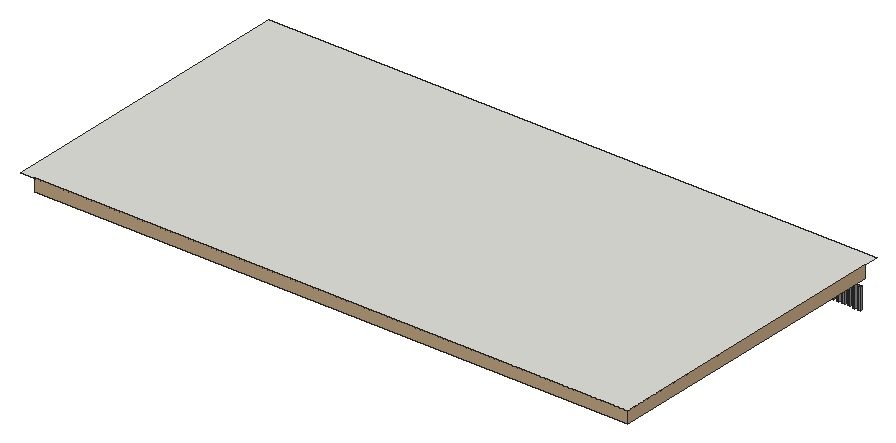
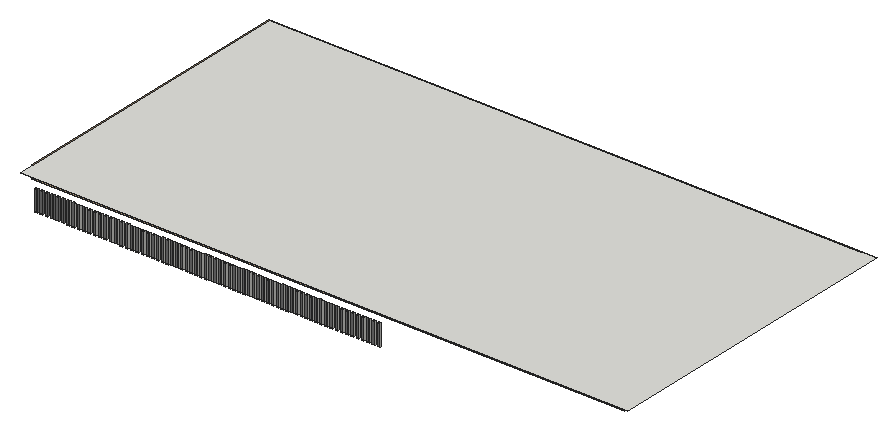
# SketchUp Ruby script. Lengths in inches.
U = 1.inch
M = Sketchup.active_model
def pt(a) = Geom::Point3d.new(a.map { |v| v * U })
def face(e, loops, mat)
  f = e.add_face(loops[0].map { |a| pt(a) })
  loops[1..].each { |l| e.add_face(l.map { |a| pt(a) }).erase! }
  f.material = f.back_material = mat if mat
  f
end
# faces: each face lists its corners as indices into pts; further lists are holes
def faces(e, pts, list, mat = nil) = list.each { |f| face(e, (f[0].is_a?(Array) ? f : [f]).map { |l| l.map { |i| pts[i] } }, mat) }
# xy, xz, yz: faces in a plane at the given z, y or x. An outline is a flat list of corners, or four numbers for a rectangle; further outlines are holes
def ring(l) = l.size == 4 ? [[l[0], l[1]], [l[2], l[1]], [l[2], l[3]], [l[0], l[3]]] : l.each_slice(2).to_a
def flat(e, list, mat, &to3) = list.each { |f| face(e, (f[0].is_a?(Array) ? f : [f]).map { |l| ring(l).map { |u, v| to3.(u, v) } }, mat) }
def xy(e, z, list, mat = nil) = flat(e, list, mat) { |x, y| [x, y, z] }
def xz(e, y, list, mat = nil) = flat(e, list, mat) { |x, z| [x, y, z] }
def yz(e, x, list, mat = nil) = flat(e, list, mat) { |y, z| [x, y, z] }
def lines(e, pts, list) = list.each { |a, b| e.add_line(pt(pts[a]), pt(pts[b])) }
# prism: a flat outline (further loops are holes) pulled along v
def prism(e, loops, v, mat = nil)
  f = face(e, loops, mat); d = Geom::Vector3d.new(v.map { |x| x * U })
  f.pushpull(f.normal.samedirection?(d) ? d.length : -d.length)
end
def box(e, o, s, mat = nil) = prism(e, [[o, [o[0] + s[0], o[1], o[2]], [o[0] + s[0], o[1] + s[1], o[2]], [o[0], o[1] + s[1], o[2]]]], [0, 0, s[2]], mat)
def at(x, y, z, deg = 0) = Geom::Transformation.translation(pt([x, y, z])) * Geom::Transformation.rotation(ORIGIN, Z_AXIS, deg.degrees)
def axes(o, x, y, z) = Geom::Transformation.new([*x, 0, *y, 0, *z, 0, *pt(o).to_a, 1])
def part(name) = M.definitions.add(name)
# library, detail: a bought-in or finely detailed component or shape, given as its bounding box
def library(name, o, s) = part(name).tap { |d| box(d.entities, o, s) }
def detail(e, o, s) = box(e.add_group.entities, o, s)
def put(e, d, t, mat = nil) = e.add_instance(d, t).tap { |i| i.material = mat if mat }
def group(e, t, mat = nil) = e.add_group.tap { |g| g.transformation = t; g.material = mat if mat }.entities
root = M.entities
M.materials.add("Maquette Wood A01 12cm").color = [209, 181, 135]
M.materials.add("Sand A01 200cm").color = [193, 166, 131]
M.materials.add("[Color M04]").color = [142, 142, 142]
c1 = library("Spot Light\#2",[-5.1,-5.1,-11.05],[10.2,10.2,11.05])
c2 = library("Spot Light\#5",[-5.1,-5.1,-11.05],[10.2,10.2,11.05])
c3 = library("Fan 90-20",[-15.86,-15.86,-9.19],[31.73,31.72,9.19])
c4 = library("Spot Light\#1",[-5.1,-5.1,-11.05],[10.2,10.2,11.05])
c5 = library("Spot Light\#6",[-5.1,-5.1,-11.05],[10.2,10.2,11.05])
c6 = library("Spot Light",[-5.1,-5.1,-11.05],[10.2,10.2,11.05])
c7 = library("Spot Light\#7",[-5.1,-5.1,-11.05],[10.2,10.2,11.05])
xy(root,222.8125,[[195.59,222.56,197.53,223.75],[199.5625,222.56,201.5,223.75],[203.53,222.56,205.47,223.75],[207.5,222.56,209.44,223.75],[211.47,222.56,213.41,223.75],
  [215.4375,222.56,217.38,223.75],[219.41,222.56,221.35,223.75],[223.38,222.56,225.32,223.75],[227.35,222.56,229.29,223.75],[231.32,222.56,233.26,223.75],
  [235.29,222.56,237.23,223.75],[239.25,222.56,241.2,223.75],[242.87,222.56,244.8125,223.75],[246.49,222.56,248.43,223.75],[250.11,222.56,252.05,223.75],
  [253.72,222.56,255.67,223.75],[257.34,222.56,259.28,223.75],[260.96,222.56,262.9,223.75],[264.58,222.56,266.52,223.75],[268.19,222.56,270.14,223.75],
  [271.8125,222.56,273.75,223.75],[275.43,222.56,277.37,223.75],[279.05,222.56,280.99,223.75],[282.66,222.56,284.61,223.75],[286.28,222.56,288.22,223.75],
  [289.9,222.56,291.84,223.75],[293.52,222.56,295.46,223.75],[297.13,222.56,299.08,223.75],[300.75,222.56,302.69,223.75],[304.37,222.56,306.31,223.75],
  [307.99,222.56,309.93,223.75],[311.6,222.56,313.55,223.75],[315.22,222.56,317.16,223.75],[318.84,222.56,320.78,223.75],[322.46,222.56,324.4,223.75],
  [326.07,222.56,328.01,223.75],[329.69,222.56,331.63,223.75],[333.31,222.56,335.25,223.75],[336.93,222.56,338.87,223.75],[340.54,222.56,342.48,223.75],
  [344.16,222.56,346.1,223.75],[347.78,222.56,349.72,223.75],[351.39,222.56,353.34,223.75],[355.01,222.56,356.95,223.75],[358.63,222.56,360.57,223.75],
  [362.44,222.56,364.38,223.75],[365.5,222.56,367.45,223.75],[369.54,222.56,371.48,223.75],[373.57,222.56,375.51,223.75],[377.6,222.56,379.54,223.75],
  [381.63,222.56,383.57,223.75],[385.66,222.56,387.6,223.75],[389.69,222.56,391.63,223.75],[393.72,222.56,395.67,223.75],[397.75,222.56,399.7,223.75],
  [401.79,222.56,403.73,223.75],[405.82,222.56,407.76,223.75],[409.85,222.56,411.79,223.75],[413.88,222.56,415.82,223.75],[417.91,222.56,419.85,223.75],
  [421.94,222.56,423.88,223.75],[425.97,222.56,427.92,223.75],[430,222.56,431.95,223.75]])
xy(root,222.8125,[[434.04,222.56,435.98,223.75],[438.07,222.56,440.01,223.75],[442.1,222.56,444.04,223.75],[446.13,222.56,448.07,223.75],[450.16,222.56,452.1,223.75],
  [454.19,222.56,456.13,223.75]],"[Color M04]")
xy(root,238.625,[[329.69,222.56,331.63,223.75],[347.78,222.56,349.72,223.75]])
xy(root,238.625,[[195.59,222.56,197.53,223.75],[199.5625,222.56,201.5,223.75],[203.53,222.56,205.47,223.75],[207.5,222.56,209.44,223.75],[211.47,222.56,213.41,223.75],
  [215.4375,222.56,217.38,223.75],[219.41,222.56,221.35,223.75],[223.38,222.56,225.32,223.75],[227.35,222.56,229.29,223.75],[231.32,222.56,233.26,223.75],
  [235.29,222.56,237.23,223.75],[239.25,222.56,241.2,223.75],[242.87,222.56,244.8125,223.75],[246.49,222.56,248.43,223.75],[250.11,222.56,252.05,223.75],
  [253.72,222.56,255.67,223.75],[257.34,222.56,259.28,223.75],[260.96,222.56,262.9,223.75],[264.58,222.56,266.52,223.75],[268.19,222.56,270.14,223.75],
  [271.8125,222.56,273.75,223.75],[275.43,222.56,277.37,223.75],[279.05,222.56,280.99,223.75],[282.66,222.56,284.61,223.75],[286.28,222.56,288.22,223.75],
  [289.9,222.56,291.84,223.75],[293.52,222.56,295.46,223.75],[297.13,222.56,299.08,223.75],[300.75,222.56,302.69,223.75],[304.37,222.56,306.31,223.75],
  [307.99,222.56,309.93,223.75],[311.6,222.56,313.55,223.75],[315.22,222.56,317.16,223.75],[318.84,222.56,320.78,223.75],[322.46,222.56,324.4,223.75],
  [326.07,222.56,328.01,223.75],[333.31,222.56,335.25,223.75],[336.93,222.56,338.87,223.75],[340.54,222.56,342.48,223.75],[344.16,222.56,346.1,223.75],
  [351.39,222.56,353.34,223.75],[355.01,222.56,356.95,223.75],[358.63,222.56,360.57,223.75],[362.44,222.56,364.38,223.75],[365.5,222.56,367.45,223.75],
  [369.54,222.56,371.48,223.75],[373.57,222.56,375.51,223.75],[377.6,222.56,379.54,223.75],[381.63,222.56,383.57,223.75],[385.66,222.56,387.6,223.75],
  [389.69,222.56,391.63,223.75],[393.72,222.56,395.67,223.75],[397.75,222.56,399.7,223.75],[401.79,222.56,403.73,223.75],[405.82,222.56,407.76,223.75],
  [409.85,222.56,411.79,223.75],[413.88,222.56,415.82,223.75],[417.91,222.56,419.85,223.75],[421.94,222.56,423.88,223.75],[425.97,222.56,427.92,223.75],
  [430,222.56,431.95,223.75],[434.04,222.56,435.98,223.75],[438.07,222.56,440.01,223.75],[442.1,222.56,444.04,223.75],[446.13,222.56,448.07,223.75],
  [450.16,222.56,452.1,223.75],[454.19,222.56,456.13,223.75]],"[Color M04]")
xy(root,240.875,[[[36.86,36.86,432.41,198.01],[119.36,152.06,123.11,152.55,126.61,154,129.61,156.31,131.92,159.31,133.37,162.81,133.86,166.56,133.37,170.3125,131.92,173.81,129.61,176.8125,126.61,179.12,123.11,180.57,119.36,181.06,115.61,180.57,112.11,179.12,109.11,176.8125,106.8,173.81,105.35,170.3125,104.86,166.56,105.35,162.81,106.8,159.31,109.11,156.31,112.11,154,115.61,152.55],[380.67,152.06,384.43,152.55,387.92,154,390.93,156.31,393.23,159.31,394.68,162.81,395.17,166.56,394.68,170.3125,393.23,173.81,390.93,176.8125,387.92,179.12,384.43,180.57,380.67,181.06,376.92,180.57,373.42,179.12,370.42,176.8125,368.12,173.81,366.67,170.3125,366.17,166.56,366.67,162.81,368.12,159.31,370.42,156.31,373.42,154,376.92,152.55],[380.67,56.94,384.43,57.43,387.92,58.88,390.93,61.18,393.23,64.19,394.68,67.68,395.17,71.44,394.68,75.1875,393.23,78.69,390.93,81.6875,387.92,83.99,384.43,85.44,380.67,85.94,376.92,85.44,373.42,83.99,370.42,81.6875,368.12,78.69,366.67,75.1875,366.17,71.44,366.67,67.68,368.12,64.19,370.42,61.18,373.42,58.88,376.92,57.43],[119.36,55.56,123.11,56.05,126.61,57.5,129.61,59.81,131.92,62.81,133.37,66.31,133.86,70.06,133.37,73.8125,131.92,77.31,129.61,80.3125,126.61,82.62,123.11,84.07,119.36,84.56,115.61,84.07,112.11,82.62,109.11,80.3125,106.8,77.31,105.35,73.8125,104.86,70.06,105.35,66.31,106.8,62.81,109.11,59.81,112.11,57.5,115.61,56.05],[286.11,152.34,288.26,152.62,290.27,153.45,291.99,154.77,293.31,156.49,294.14,158.5,294.42,160.65,294.14,162.8,293.31,164.8,291.99,166.53,290.27,167.85,288.26,168.68,286.11,168.96,283.96,168.68,281.95,167.85,280.23,166.53,278.91,164.8,278.08,162.8,277.8,160.65,278.08,158.5,278.91,156.49,280.23,154.77,281.95,153.45,283.96,152.62],[201.74,152.34,203.89,152.62,205.89,153.45,207.61,154.77,208.93,156.49,209.76,158.5,210.05,160.65,209.76,162.8,208.93,164.8,207.61,166.53,205.89,167.85,203.89,168.68,201.74,168.96,199.58,168.68,197.58,167.85,195.86,166.53,194.54,164.8,193.71,162.8,193.42,160.65,193.71,158.5,194.54,156.49,195.86,154.77,197.58,153.45,199.58,152.62],[201.74,60.65,203.89,60.93,205.89,61.76,207.61,63.08,208.93,64.8,209.76,66.81,210.05,68.96,209.76,71.11,208.93,73.12,207.61,74.84,205.89,76.16,203.89,76.99,201.74,77.27,199.58,76.99,197.58,76.16,195.86,74.84,194.54,73.12,193.71,71.11,193.42,68.96,193.71,66.81,194.54,64.8,195.86,63.08,197.58,61.76,199.58,60.93],[286.11,63.4,288.26,63.68,290.27,64.51,291.99,65.83,293.31,67.55,294.14,69.56,294.42,71.71,294.14,73.86,293.31,75.87,291.99,77.59,290.27,78.91,288.26,79.74,286.11,80.02,283.96,79.74,281.95,78.91,280.23,77.59,278.91,75.87,278.08,73.86,277.8,71.71,278.08,69.56,278.91,67.55,280.23,65.83,281.95,64.51,283.96,63.68]]],"[Color M04]")
xy(root,242.375,[[286.11,63.4,283.96,63.68,281.95,64.51,280.23,65.83,278.91,67.55,278.08,69.56,277.8,71.71,278.08,73.86,278.91,75.87,280.23,77.59,281.95,78.91,283.96,79.74,286.11,80.02,288.26,79.74,290.27,78.91,291.99,77.59,293.31,75.87,294.14,73.86,294.42,71.71,294.14,69.56,293.31,67.55,291.99,65.83,290.27,64.51,288.26,63.68]],"[Color M04]")
xy(root,242.5625,[[201.74,60.65,199.58,60.93,197.58,61.76,195.86,63.08,194.54,64.8,193.71,66.81,193.42,68.96,193.71,71.11,194.54,73.12,195.86,74.84,197.58,76.16,199.58,76.99,201.74,77.27,203.89,76.99,205.89,76.16,207.61,74.84,208.93,73.12,209.76,71.11,210.05,68.96,209.76,66.81,208.93,64.8,207.61,63.08,205.89,61.76,203.89,60.93]],"[Color M04]")
xy(root,242.75,[[201.74,152.34,199.58,152.62,197.58,153.45,195.86,154.77,194.54,156.49,193.71,158.5,193.42,160.65,193.71,162.8,194.54,164.8,195.86,166.53,197.58,167.85,199.58,168.68,201.74,168.96,203.89,168.68,205.89,167.85,207.61,166.53,208.93,164.8,209.76,162.8,210.05,160.65,209.76,158.5,208.93,156.49,207.61,154.77,205.89,153.45,203.89,152.62]],"[Color M04]")
xy(root,242.875,[[286.11,152.34,283.96,152.62,281.95,153.45,280.23,154.77,278.91,156.49,278.08,158.5,277.8,160.65,278.08,162.8,278.91,164.8,280.23,166.53,281.95,167.85,283.96,168.68,286.11,168.96,288.26,168.68,290.27,167.85,291.99,166.53,293.31,164.8,294.14,162.8,294.42,160.65,294.14,158.5,293.31,156.49,291.99,154.77,290.27,153.45,288.26,152.62]],"[Color M04]")
xy(root,242.9375,[[380.67,152.06,376.92,152.55,373.42,154,370.42,156.31,368.12,159.31,366.67,162.81,366.17,166.56,366.67,170.3125,368.12,173.81,370.42,176.8125,373.42,179.12,376.92,180.57,380.67,181.06,384.43,180.57,387.92,179.12,390.93,176.8125,393.23,173.81,394.68,170.3125,395.17,166.56,394.68,162.81,393.23,159.31,390.93,156.31,387.92,154,384.43,152.55]],"[Color M04]")
xy(root,243.0625,[[380.67,56.94,376.92,57.43,373.42,58.88,370.42,61.18,368.12,64.19,366.67,67.68,366.17,71.44,366.67,75.1875,368.12,78.69,370.42,81.6875,373.42,83.99,376.92,85.44,380.67,85.94,384.43,85.44,387.92,83.99,390.93,81.6875,393.23,78.69,394.68,75.1875,395.17,71.44,394.68,67.68,393.23,64.19,390.93,61.18,387.92,58.88,384.43,57.43]],"[Color M04]")
xy(root,244.625,[[[31.46,31.46,437.81,203.41],[36.86,36.86,432.41,198.01]]],"Maquette Wood A01 12cm")
xy(root,244.625,[[[11.13,11.13,458.14,223.75],[31.46,31.46,437.81,203.41]]],"Sand A01 200cm")
xy(root,253.625,[[0,0,458.14,234.875]])
xz(root,0,[[11.13,244.625,458.14,253.625]],"Sand A01 200cm")
xz(root,36.86,[[36.86,240.875,432.41,244.625]],"[Color M04]")
xz(root,198.01,[[36.86,240.875,432.41,244.625]],"[Color M04]")
xz(root,222.56,[[195.59,222.8125,197.53,238.625],[199.5625,222.8125,201.5,238.625],[203.53,222.8125,205.47,238.625],[207.5,222.8125,209.44,238.625],[211.47,222.8125,213.41,238.625],
  [215.4375,222.8125,217.38,238.625],[219.41,222.8125,221.35,238.625],[223.38,222.8125,225.32,238.625],[227.35,222.8125,229.29,238.625],[231.32,222.8125,233.26,238.625],
  [235.29,222.8125,237.23,238.625],[239.25,222.8125,241.2,238.625],[242.87,222.8125,244.8125,238.625],[246.49,222.8125,248.43,238.625],[250.11,222.8125,252.05,238.625],
  [253.72,222.8125,255.67,238.625],[257.34,222.8125,259.28,238.625],[260.96,222.8125,262.9,238.625],[264.58,222.8125,266.52,238.625],[268.19,222.8125,270.14,238.625],
  [271.8125,222.8125,273.75,238.625],[275.43,222.8125,277.37,238.625],[279.05,222.8125,280.99,238.625],[282.66,222.8125,284.61,238.625],[286.28,222.8125,288.22,238.625],
  [289.9,222.8125,291.84,238.625],[293.52,222.8125,295.46,238.625],[297.13,222.8125,299.08,238.625],[300.75,222.8125,302.69,238.625],[304.37,222.8125,306.31,238.625],
  [307.99,222.8125,309.93,238.625],[311.6,222.8125,313.55,238.625],[315.22,222.8125,317.16,238.625],[318.84,222.8125,320.78,238.625],[322.46,222.8125,324.4,238.625],
  [326.07,222.8125,328.01,238.625],[329.69,222.8125,331.63,238.625],[333.31,222.8125,335.25,238.625],[336.93,222.8125,338.87,238.625],[340.54,222.8125,342.48,238.625],
  [344.16,222.8125,346.1,238.625],[347.78,222.8125,349.72,238.625],[351.39,222.8125,353.34,238.625],[355.01,222.8125,356.95,238.625],[358.63,222.8125,360.57,238.625],
  [362.44,222.8125,364.38,238.625],[365.5,222.8125,367.45,238.625],[369.54,222.8125,371.48,238.625],[373.57,222.8125,375.51,238.625],[377.6,222.8125,379.54,238.625],
  [381.63,222.8125,383.57,238.625],[385.66,222.8125,387.6,238.625],[389.69,222.8125,391.63,238.625],[393.72,222.8125,395.67,238.625],[397.75,222.8125,399.7,238.625],
  [401.79,222.8125,403.73,238.625],[405.82,222.8125,407.76,238.625],[409.85,222.8125,411.79,238.625],[413.88,222.8125,415.82,238.625],[417.91,222.8125,419.85,238.625],
  [421.94,222.8125,423.88,238.625],[425.97,222.8125,427.92,238.625],[430,222.8125,431.95,238.625],[434.04,222.8125,435.98,238.625],[438.07,222.8125,440.01,238.625],
  [442.1,222.8125,444.04,238.625],[446.13,222.8125,448.07,238.625],[450.16,222.8125,452.1,238.625],[454.19,222.8125,456.13,238.625]],"[Color M04]")
yz(root,195.59,[[222.56,222.8125,223.75,238.625]])
yz(root,197.53,[[222.56,222.8125,223.75,238.625]],"[Color M04]")
yz(root,199.5625,[[222.56,222.8125,223.75,238.625]])
yz(root,201.5,[[222.56,222.8125,223.75,238.625]],"[Color M04]")
yz(root,203.53,[[222.56,222.8125,223.75,238.625]])
yz(root,205.47,[[222.56,222.8125,223.75,238.625]],"[Color M04]")
yz(root,207.5,[[222.56,222.8125,223.75,238.625]])
yz(root,209.44,[[222.56,222.8125,223.75,238.625]],"[Color M04]")
yz(root,211.47,[[222.56,222.8125,223.75,238.625]])
yz(root,213.41,[[222.56,222.8125,223.75,238.625]],"[Color M04]")
yz(root,215.4375,[[222.56,222.8125,223.75,238.625]])
yz(root,217.38,[[222.56,222.8125,223.75,238.625]],"[Color M04]")
yz(root,219.41,[[222.56,222.8125,223.75,238.625]])
yz(root,221.35,[[222.56,222.8125,223.75,238.625]],"[Color M04]")
yz(root,223.38,[[222.56,222.8125,223.75,238.625]])
yz(root,225.32,[[222.56,222.8125,223.75,238.625]],"[Color M04]")
yz(root,227.35,[[222.56,222.8125,223.75,238.625]])
yz(root,229.29,[[222.56,222.8125,223.75,238.625]],"[Color M04]")
yz(root,231.32,[[222.56,222.8125,223.75,238.625]])
yz(root,233.26,[[222.56,222.8125,223.75,238.625]],"[Color M04]")
yz(root,235.29,[[222.56,222.8125,223.75,238.625]])
yz(root,237.23,[[222.56,222.8125,223.75,238.625]],"[Color M04]")
yz(root,239.25,[[222.56,222.8125,223.75,238.625]])
yz(root,241.2,[[222.56,222.8125,223.75,238.625]],"[Color M04]")
yz(root,242.87,[[222.56,222.8125,223.75,238.625]])
yz(root,244.8125,[[222.56,222.8125,223.75,238.625]],"[Color M04]")
yz(root,246.49,[[222.56,222.8125,223.75,238.625]])
yz(root,248.43,[[222.56,222.8125,223.75,238.625]],"[Color M04]")
yz(root,250.11,[[222.56,222.8125,223.75,238.625]])
yz(root,252.05,[[222.56,222.8125,223.75,238.625]],"[Color M04]")
yz(root,253.72,[[222.56,222.8125,223.75,238.625]])
yz(root,255.67,[[222.56,222.8125,223.75,238.625]],"[Color M04]")
yz(root,257.34,[[222.56,222.8125,223.75,238.625]])
yz(root,259.28,[[222.56,222.8125,223.75,238.625]],"[Color M04]")
yz(root,260.96,[[222.56,222.8125,223.75,238.625]])
yz(root,262.9,[[222.56,222.8125,223.75,238.625]],"[Color M04]")
yz(root,264.58,[[222.56,222.8125,223.75,238.625]])
yz(root,266.52,[[222.56,222.8125,223.75,238.625]],"[Color M04]")
yz(root,268.19,[[222.56,222.8125,223.75,238.625]])
yz(root,270.14,[[222.56,222.8125,223.75,238.625]],"[Color M04]")
yz(root,271.8125,[[222.56,222.8125,223.75,238.625]])
yz(root,273.75,[[222.56,222.8125,223.75,238.625]],"[Color M04]")
yz(root,275.43,[[222.56,222.8125,223.75,238.625]])
yz(root,277.37,[[222.56,222.8125,223.75,238.625]],"[Color M04]")
yz(root,279.05,[[222.56,222.8125,223.75,238.625]])
yz(root,280.99,[[222.56,222.8125,223.75,238.625]],"[Color M04]")
yz(root,282.66,[[222.56,222.8125,223.75,238.625]])
yz(root,284.61,[[222.56,222.8125,223.75,238.625]],"[Color M04]")
yz(root,286.28,[[222.56,222.8125,223.75,238.625]])
yz(root,288.22,[[222.56,222.8125,223.75,238.625]],"[Color M04]")
yz(root,289.9,[[222.56,222.8125,223.75,238.625]])
yz(root,291.84,[[222.56,222.8125,223.75,238.625]],"[Color M04]")
yz(root,293.52,[[222.56,222.8125,223.75,238.625]])
yz(root,295.46,[[222.56,222.8125,223.75,238.625]],"[Color M04]")
yz(root,297.13,[[222.56,222.8125,223.75,238.625]])
yz(root,299.08,[[222.56,222.8125,223.75,238.625]],"[Color M04]")
yz(root,300.75,[[222.56,222.8125,223.75,238.625]])
yz(root,302.69,[[222.56,222.8125,223.75,238.625]],"[Color M04]")
yz(root,304.37,[[222.56,222.8125,223.75,238.625]])
yz(root,306.31,[[222.56,222.8125,223.75,238.625]],"[Color M04]")
yz(root,307.99,[[222.56,222.8125,223.75,238.625]])
yz(root,309.93,[[222.56,222.8125,223.75,238.625]],"[Color M04]")
yz(root,311.6,[[222.56,222.8125,223.75,238.625]])
yz(root,313.55,[[222.56,222.8125,223.75,238.625]],"[Color M04]")
yz(root,315.22,[[222.56,222.8125,223.75,238.625]])
yz(root,317.16,[[222.56,222.8125,223.75,238.625]],"[Color M04]")
yz(root,318.84,[[222.56,222.8125,223.75,238.625]])
yz(root,320.78,[[222.56,222.8125,223.75,238.625]],"[Color M04]")
yz(root,322.46,[[222.56,222.8125,223.75,238.625]])
yz(root,324.4,[[222.56,222.8125,223.75,238.625]],"[Color M04]")
yz(root,326.07,[[222.56,222.8125,223.75,238.625]])
yz(root,328.01,[[222.56,222.8125,223.75,238.625]],"[Color M04]")
yz(root,329.69,[[222.56,222.8125,223.75,238.625]])
yz(root,331.63,[[222.56,222.8125,223.75,238.625]],"[Color M04]")
yz(root,333.31,[[222.56,222.8125,223.75,238.625]])
yz(root,335.25,[[222.56,222.8125,223.75,238.625]],"[Color M04]")
yz(root,336.93,[[222.56,222.8125,223.75,238.625]])
yz(root,338.87,[[222.56,222.8125,223.75,238.625]],"[Color M04]")
yz(root,340.54,[[222.56,222.8125,223.75,238.625]])
yz(root,342.48,[[222.56,222.8125,223.75,238.625]],"[Color M04]")
yz(root,344.16,[[222.56,222.8125,223.75,238.625]])
yz(root,346.1,[[222.56,222.8125,223.75,238.625]],"[Color M04]")
yz(root,347.78,[[222.56,222.8125,223.75,238.625]])
yz(root,349.72,[[222.56,222.8125,223.75,238.625]],"[Color M04]")
yz(root,351.39,[[222.56,222.8125,223.75,238.625]])
yz(root,353.34,[[222.56,222.8125,223.75,238.625]],"[Color M04]")
yz(root,355.01,[[222.56,222.8125,223.75,238.625]])
yz(root,356.95,[[222.56,222.8125,223.75,238.625]],"[Color M04]")
yz(root,358.63,[[222.56,222.8125,223.75,238.625]])
yz(root,360.57,[[222.56,222.8125,223.75,238.625]],"[Color M04]")
yz(root,362.44,[[222.56,222.8125,223.75,238.625]])
yz(root,364.38,[[222.56,222.8125,223.75,238.625]],"[Color M04]")
yz(root,365.5,[[222.56,222.8125,223.75,238.625]])
yz(root,367.45,[[222.56,222.8125,223.75,238.625]],"[Color M04]")
yz(root,369.54,[[222.56,222.8125,223.75,238.625]])
yz(root,371.48,[[222.56,222.8125,223.75,238.625]],"[Color M04]")
yz(root,373.57,[[222.56,222.8125,223.75,238.625]])
yz(root,375.51,[[222.56,222.8125,223.75,238.625]],"[Color M04]")
yz(root,377.6,[[222.56,222.8125,223.75,238.625]])
yz(root,379.54,[[222.56,222.8125,223.75,238.625]],"[Color M04]")
yz(root,381.63,[[222.56,222.8125,223.75,238.625]])
yz(root,383.57,[[222.56,222.8125,223.75,238.625]],"[Color M04]")
yz(root,385.66,[[222.56,222.8125,223.75,238.625]])
yz(root,387.6,[[222.56,222.8125,223.75,238.625]],"[Color M04]")
yz(root,389.69,[[222.56,222.8125,223.75,238.625]])
yz(root,391.63,[[222.56,222.8125,223.75,238.625]],"[Color M04]")
yz(root,393.72,[[222.56,222.8125,223.75,238.625]])
yz(root,395.67,[[222.56,222.8125,223.75,238.625]],"[Color M04]")
yz(root,397.75,[[222.56,222.8125,223.75,238.625]])
yz(root,399.7,[[222.56,222.8125,223.75,238.625]],"[Color M04]")
yz(root,401.79,[[222.56,222.8125,223.75,238.625]])
yz(root,403.73,[[222.56,222.8125,223.75,238.625]],"[Color M04]")
yz(root,405.82,[[222.56,222.8125,223.75,238.625]])
yz(root,407.76,[[222.56,222.8125,223.75,238.625]],"[Color M04]")
yz(root,409.85,[[222.56,222.8125,223.75,238.625]])
yz(root,411.79,[[222.56,222.8125,223.75,238.625]],"[Color M04]")
yz(root,413.88,[[222.56,222.8125,223.75,238.625]])
yz(root,415.82,[[222.56,222.8125,223.75,238.625]],"[Color M04]")
yz(root,417.91,[[222.56,222.8125,223.75,238.625]])
yz(root,419.85,[[222.56,222.8125,223.75,238.625]],"[Color M04]")
yz(root,421.94,[[222.56,222.8125,223.75,238.625]])
yz(root,423.88,[[222.56,222.8125,223.75,238.625]],"[Color M04]")
yz(root,425.97,[[222.56,222.8125,223.75,238.625]])
yz(root,427.92,[[222.56,222.8125,223.75,238.625]],"[Color M04]")
yz(root,430,[[222.56,222.8125,223.75,238.625]])
yz(root,431.95,[[222.56,222.8125,223.75,238.625]],"[Color M04]")
yz(root,432.41,[[36.86,240.875,198.01,244.625]],"[Color M04]")
yz(root,434.04,[[222.56,222.8125,223.75,238.625]],"[Color M04]")
yz(root,435.98,[[222.56,222.8125,223.75,238.625]],"[Color M04]")
yz(root,438.07,[[222.56,222.8125,223.75,238.625]],"[Color M04]")
yz(root,440.01,[[222.56,222.8125,223.75,238.625]],"[Color M04]")
yz(root,442.1,[[222.56,222.8125,223.75,238.625]],"[Color M04]")
yz(root,444.04,[[222.56,222.8125,223.75,238.625]],"[Color M04]")
yz(root,446.13,[[222.56,222.8125,223.75,238.625]],"[Color M04]")
yz(root,448.07,[[222.56,222.8125,223.75,238.625]],"[Color M04]")
yz(root,450.16,[[222.56,222.8125,223.75,238.625]],"[Color M04]")
yz(root,452.1,[[222.56,222.8125,223.75,238.625]],"[Color M04]")
yz(root,454.19,[[222.56,222.8125,223.75,238.625]],"[Color M04]")
yz(root,456.13,[[222.56,222.8125,223.75,238.625]],"[Color M04]")
yz(root,458.14,[[0,244.625,223.75,253.625]],"Sand A01 200cm")
p = [[380.67,56.94,240.875],[376.92,57.43,240.875],[376.92,57.43,243.0625],[380.67,56.94,243.0625],[384.43,57.43,240.875],[384.43,57.43,243.0625],
  [373.42,58.88,240.875],[373.42,58.88,243.0625],[387.92,58.88,240.875],[387.92,58.88,243.0625],[370.42,61.18,240.875],[370.42,61.18,243.0625],
  [390.93,61.18,240.875],[390.93,61.18,243.0625],[201.74,60.65,240.875],[199.58,60.93,240.875],[199.58,60.93,242.5625],[201.74,60.65,242.5625],
  [203.89,60.93,240.875],[203.89,60.93,242.5625],[197.58,61.76,240.875],[197.58,61.76,242.5625],[205.89,61.76,240.875],[205.89,61.76,242.5625],
  [368.12,64.19,240.875],[368.12,64.19,243.0625],[393.23,64.19,240.875],[393.23,64.19,243.0625],[195.86,63.08,240.875],[195.86,63.08,242.5625],
  [207.61,63.08,240.875],[207.61,63.08,242.5625],[194.54,64.8,240.875],[194.54,64.8,242.5625],[208.93,64.8,240.875],[208.93,64.8,242.5625],
  [286.11,63.4,240.875],[283.96,63.68,240.875],[283.96,63.68,242.375],[286.11,63.4,242.375],[288.26,63.68,240.875],[288.26,63.68,242.375],
  [281.95,64.51,240.875],[281.95,64.51,242.375],[290.27,64.51,240.875],[290.27,64.51,242.375],[366.67,67.68,240.875],[366.67,67.68,243.0625],
  [394.68,67.68,240.875],[394.68,67.68,243.0625],[280.23,65.83,240.875],[280.23,65.83,242.375],[291.99,65.83,240.875],[291.99,65.83,242.375],
  [193.71,66.81,240.875],[193.71,66.81,242.5625],[209.76,66.81,240.875],[209.76,66.81,242.5625],[278.91,67.55,240.875],[278.91,67.55,242.375],
  [293.31,67.55,240.875],[293.31,67.55,242.375],[210.05,68.96,240.875],[210.05,68.96,242.5625],[278.08,69.56,240.875],[278.08,69.56,242.375],
  [294.14,69.56,240.875],[294.14,69.56,242.375],[366.17,71.44,240.875],[366.17,71.44,243.0625],[395.17,71.44,240.875],[395.17,71.44,243.0625],
  [209.76,71.11,240.875],[209.76,71.11,242.5625],[277.8,71.71,240.875],[277.8,71.71,242.375],[294.42,71.71,240.875],[294.42,71.71,242.375],
  [193.71,71.11,240.875],[194.54,73.12,240.875],[194.54,73.12,242.5625],[193.71,71.11,242.5625],[208.93,73.12,240.875],[208.93,73.12,242.5625],
  [366.67,75.1875,240.875],[366.67,75.1875,243.0625],[394.68,75.1875,240.875],[394.68,75.1875,243.0625],[278.08,73.86,240.875],[278.08,73.86,242.375],
  [294.14,73.86,240.875],[294.14,73.86,242.375],[195.86,74.84,240.875],[195.86,74.84,242.5625],[207.61,74.84,240.875],[207.61,74.84,242.5625],
  [278.91,75.87,240.875],[278.91,75.87,242.375],[293.31,75.87,240.875],[293.31,75.87,242.375],[197.58,76.16,240.875],[197.58,76.16,242.5625],
  [205.89,76.16,240.875],[205.89,76.16,242.5625],[368.12,78.69,240.875],[368.12,78.69,243.0625],[393.23,78.69,240.875],[393.23,78.69,243.0625],
  [280.23,77.59,240.875],[280.23,77.59,242.375],[291.99,77.59,240.875],[291.99,77.59,242.375],[199.58,76.99,240.875],[199.58,76.99,242.5625],
  [203.89,76.99,240.875],[203.89,76.99,242.5625],[201.74,77.27,240.875],[201.74,77.27,242.5625],[281.95,78.91,240.875],[281.95,78.91,242.375],
  [290.27,78.91,240.875],[290.27,78.91,242.375],[370.42,81.6875,240.875],[370.42,81.6875,243.0625],[390.93,81.6875,240.875],[390.93,81.6875,243.0625],
  [283.96,79.74,240.875],[283.96,79.74,242.375],[288.26,79.74,240.875],[288.26,79.74,242.375],[286.11,80.02,240.875],[286.11,80.02,242.375],
  [373.42,83.99,240.875],[373.42,83.99,243.0625],[387.92,83.99,240.875],[387.92,83.99,243.0625],[376.92,85.44,240.875],[376.92,85.44,243.0625],
  [384.43,85.44,240.875],[384.43,85.44,243.0625],[380.67,85.94,240.875],[380.67,85.94,243.0625],[380.67,152.06,240.875],[376.92,152.55,240.875],
  [376.92,152.55,242.9375],[380.67,152.06,242.9375],[384.43,152.55,240.875],[384.43,152.55,242.9375],[201.74,152.34,240.875],[199.58,152.62,240.875],
  [199.58,152.62,242.75],[201.74,152.34,242.75],[203.89,152.62,240.875],[203.89,152.62,242.75],[286.11,152.34,240.875],[283.96,152.62,240.875],
  [283.96,152.62,242.875],[286.11,152.34,242.875],[288.26,152.62,240.875],[288.26,152.62,242.875],[197.58,153.45,240.875],[197.58,153.45,242.75],
  [205.89,153.45,240.875],[205.89,153.45,242.75],[281.95,153.45,240.875],[281.95,153.45,242.875],[290.27,153.45,240.875],[290.27,153.45,242.875],
  [373.42,154,240.875],[373.42,154,242.9375],[387.92,154,240.875],[387.92,154,242.9375],[195.86,154.77,240.875],[195.86,154.77,242.75],
  [207.61,154.77,240.875],[207.61,154.77,242.75],[280.23,154.77,240.875],[280.23,154.77,242.875],[291.99,154.77,240.875],[291.99,154.77,242.875],
  [370.42,156.31,240.875],[370.42,156.31,242.9375],[390.93,156.31,240.875],[390.93,156.31,242.9375],[194.54,156.49,240.875],[194.54,156.49,242.75],
  [208.93,156.49,240.875],[208.93,156.49,242.75],[278.91,156.49,240.875],[278.91,156.49,242.875],[293.31,156.49,240.875],[293.31,156.49,242.875],
  [368.12,159.31,240.875],[368.12,159.31,242.9375],[393.23,159.31,240.875],[393.23,159.31,242.9375],[193.71,158.5,240.875],[193.71,158.5,242.75],
  [209.76,158.5,240.875],[209.76,158.5,242.75],[278.08,158.5,240.875],[278.08,158.5,242.875],[294.14,158.5,240.875],[294.14,158.5,242.875],
  [210.05,160.65,240.875],[210.05,160.65,242.75],[277.8,160.65,240.875],[277.8,160.65,242.875],[294.42,160.65,240.875],[294.42,160.65,242.875],
  [366.67,162.81,240.875],[366.67,162.81,242.9375],[394.68,162.81,240.875],[394.68,162.81,242.9375],[209.76,162.8,240.875],[209.76,162.8,242.75],
  [278.08,162.8,240.875],[278.08,162.8,242.875],[294.14,162.8,240.875],[294.14,162.8,242.875],[193.71,162.8,240.875],[194.54,164.8,240.875],
  [194.54,164.8,242.75],[193.71,162.8,242.75],[208.93,164.8,240.875],[208.93,164.8,242.75],[278.91,164.8,240.875],[278.91,164.8,242.875],
  [293.31,164.8,240.875],[293.31,164.8,242.875],[366.17,166.56,240.875],[366.17,166.56,242.9375],[395.17,166.56,240.875],[395.17,166.56,242.9375],
  [195.86,166.53,240.875],[195.86,166.53,242.75],[207.61,166.53,240.875],[207.61,166.53,242.75],[280.23,166.53,240.875],[280.23,166.53,242.875],
  [291.99,166.53,240.875],[291.99,166.53,242.875],[197.58,167.85,240.875],[197.58,167.85,242.75],[205.89,167.85,240.875],[205.89,167.85,242.75],
  [281.95,167.85,240.875],[281.95,167.85,242.875],[290.27,167.85,240.875],[290.27,167.85,242.875],[366.67,170.3125,240.875],[366.67,170.3125,242.9375],
  [394.68,170.3125,240.875],[394.68,170.3125,242.9375],[199.58,168.68,240.875],[199.58,168.68,242.75],[203.89,168.68,240.875],[203.89,168.68,242.75],
  [283.96,168.68,240.875],[283.96,168.68,242.875],[288.26,168.68,240.875],[288.26,168.68,242.875],[201.74,168.96,240.875],[201.74,168.96,242.75],
  [286.11,168.96,240.875],[286.11,168.96,242.875],[368.12,173.81,240.875],[368.12,173.81,242.9375],[393.23,173.81,240.875],[393.23,173.81,242.9375],
  [370.42,176.8125,240.875],[370.42,176.8125,242.9375],[390.93,176.8125,240.875],[390.93,176.8125,242.9375],[373.42,179.12,240.875],[373.42,179.12,242.9375],
  [387.92,179.12,240.875],[387.92,179.12,242.9375],[376.92,180.57,240.875],[376.92,180.57,242.9375],[384.43,180.57,240.875],[384.43,180.57,242.9375],
  [380.67,181.06,240.875],[380.67,181.06,242.9375]]
faces(root,p,[[0,1,2,3],[4,0,3,5],[1,6,7,2],[8,4,5,9],[6,10,11,7],[12,8,9,13],[14,15,16,17],[18,14,17,19],
  [15,20,21,16],[22,18,19,23],[10,24,25,11],[26,12,13,27],[20,28,29,21],[30,22,23,31],[28,32,33,29],[34,30,31,35],
  [36,37,38,39],[40,36,39,41],[37,42,43,38],[44,40,41,45],[24,46,47,25],[48,26,27,49],[42,50,51,43],[52,44,45,53],
  [32,54,55,33],[56,34,35,57],[50,58,59,51],[60,52,53,61],[62,56,57,63],[58,64,65,59],[66,60,61,67],[46,68,69,47],
  [70,48,49,71],[72,62,63,73],[64,74,75,65],[76,66,67,77],[78,79,80,81],[82,72,73,83],[68,84,85,69],[86,70,71,87],
  [74,88,89,75],[90,76,77,91],[79,92,93,80],[94,82,83,95],[88,96,97,89],[98,90,91,99],[92,100,101,93],[102,94,95,103],
  [84,104,105,85],[106,86,87,107],[96,108,109,97],[110,98,99,111],[100,112,113,101],[114,102,103,115],[112,116,117,113],[116,114,115,117],
  [108,118,119,109],[120,110,111,121],[104,122,123,105],[124,106,107,125],[118,126,127,119],[128,120,121,129],[126,130,131,127],[130,128,129,131],
  [122,132,133,123],[134,124,125,135],[132,136,137,133],[138,134,135,139],[136,140,141,137],[140,138,139,141],[142,143,144,145],[146,142,145,147],
  [148,149,150,151],[152,148,151,153],[154,155,156,157],[158,154,157,159],[149,160,161,150],[162,152,153,163],[155,164,165,156],[166,158,159,167],
  [143,168,169,144],[170,146,147,171],[160,172,173,161],[174,162,163,175],[164,176,177,165],[178,166,167,179],[168,180,181,169],[182,170,171,183],
  [172,184,185,173],[186,174,175,187],[176,188,189,177],[190,178,179,191],[180,192,193,181],[194,182,183,195],[184,196,197,185],[198,186,187,199],
  [188,200,201,189],[202,190,191,203],[204,198,199,205],[200,206,207,201],[208,202,203,209],[192,210,211,193],[212,194,195,213],[214,204,205,215],
  [206,216,217,207],[218,208,209,219],[220,221,222,223],[224,214,215,225],[216,226,227,217],[228,218,219,229],[210,230,231,211],[232,212,213,233],
  [221,234,235,222],[236,224,225,237],[226,238,239,227],[240,228,229,241],[234,242,243,235],[244,236,237,245],[238,246,247,239],[248,240,241,249],
  [230,250,251,231],[252,232,233,253],[242,254,255,243],[256,244,245,257],[246,258,259,247],[260,248,249,261],[254,262,263,255],[262,256,257,263],
  [258,264,265,259],[264,260,261,265],[250,266,267,251],[268,252,253,269],[266,270,271,267],[272,268,269,273],[270,274,275,271],[276,272,273,277],
  [274,278,279,275],[280,276,277,281],[278,282,283,279],[282,280,281,283]],"[Color M04]")
put(root,c1,at(201.74,69.56,237.11))
put(root,c2,at(201.74,161.49,238.93))
put(root,c3,axes([212.14,115.28,240.875],[1.5594,0,0],[0,1.5594,0],[0,0,1.5594]))
put(root,c4,at(286.11,71.34,236.5))
put(root,c5,at(286.11,160.32,238.49))
put(root,c3,axes([371.8,120.85,240.875],[1.5594,0,0],[0,1.5594,0],[0,0,1.5594]))
put(root,c6,at(380.67,71.43,237.21))
put(root,c7,at(380.67,168.06,238.55))
